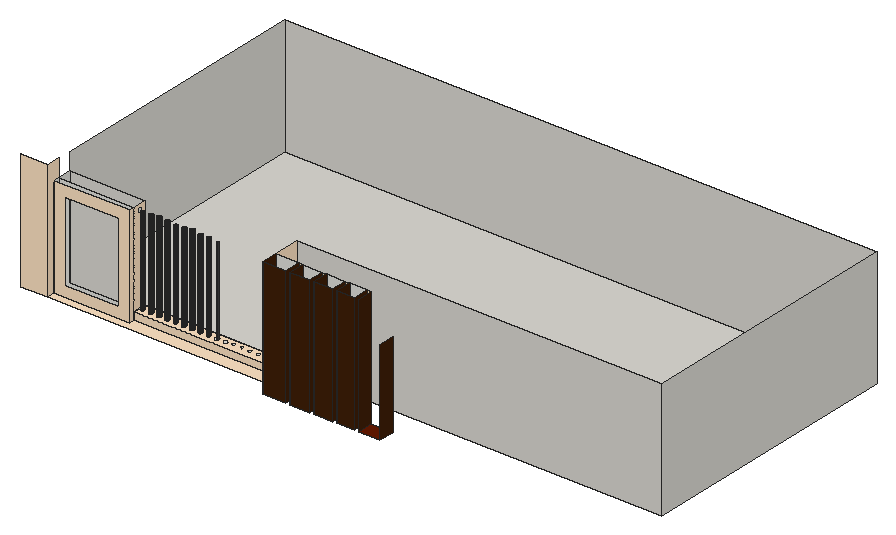
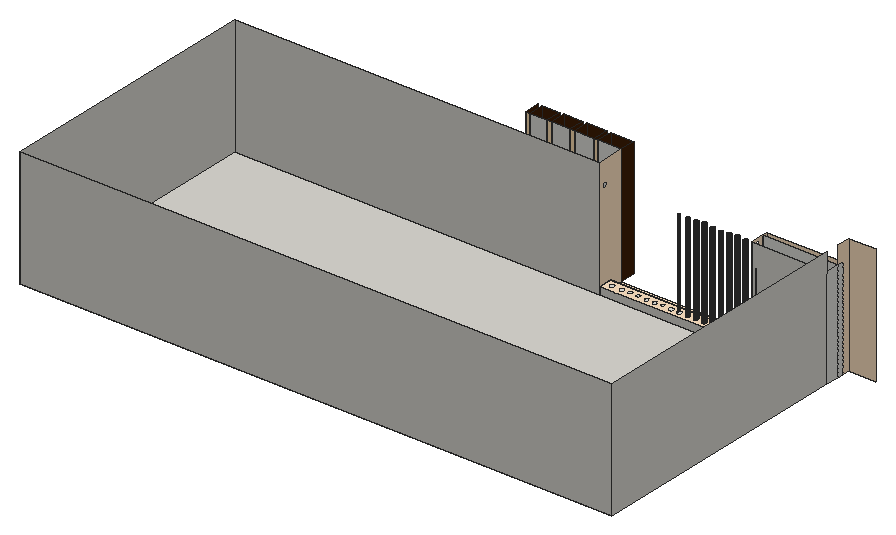
# SketchUp Ruby script. Lengths in inches.
U = 1.inch
M = Sketchup.active_model
def pt(a) = Geom::Point3d.new(a.map { |v| v * U })
def face(e, loops, mat)
  f = e.add_face(loops[0].map { |a| pt(a) })
  loops[1..].each { |l| e.add_face(l.map { |a| pt(a) }).erase! }
  f.material = f.back_material = mat if mat
  f
end
# faces: each face lists its corners as indices into pts; further lists are holes
def faces(e, pts, list, mat = nil) = list.each { |f| face(e, (f[0].is_a?(Array) ? f : [f]).map { |l| l.map { |i| pts[i] } }, mat) }
# xy, xz, yz: faces in a plane at the given z, y or x. An outline is a flat list of corners, or four numbers for a rectangle; further outlines are holes
def ring(l) = l.size == 4 ? [[l[0], l[1]], [l[2], l[1]], [l[2], l[3]], [l[0], l[3]]] : l.each_slice(2).to_a
def flat(e, list, mat, &to3) = list.each { |f| face(e, (f[0].is_a?(Array) ? f : [f]).map { |l| ring(l).map { |u, v| to3.(u, v) } }, mat) }
def xy(e, z, list, mat = nil) = flat(e, list, mat) { |x, y| [x, y, z] }
def xz(e, y, list, mat = nil) = flat(e, list, mat) { |x, z| [x, y, z] }
def yz(e, x, list, mat = nil) = flat(e, list, mat) { |y, z| [x, y, z] }
def lines(e, pts, list) = list.each { |a, b| e.add_line(pt(pts[a]), pt(pts[b])) }
# prism: a flat outline (further loops are holes) pulled along v
def prism(e, loops, v, mat = nil)
  f = face(e, loops, mat); d = Geom::Vector3d.new(v.map { |x| x * U })
  f.pushpull(f.normal.samedirection?(d) ? d.length : -d.length)
end
def box(e, o, s, mat = nil) = prism(e, [[o, [o[0] + s[0], o[1], o[2]], [o[0] + s[0], o[1] + s[1], o[2]], [o[0], o[1] + s[1], o[2]]]], [0, 0, s[2]], mat)
def at(x, y, z, deg = 0) = Geom::Transformation.translation(pt([x, y, z])) * Geom::Transformation.rotation(ORIGIN, Z_AXIS, deg.degrees)
def axes(o, x, y, z) = Geom::Transformation.new([*x, 0, *y, 0, *z, 0, *pt(o).to_a, 1])
def part(name) = M.definitions.add(name)
# library, detail: a bought-in or finely detailed component or shape, given as its bounding box
def library(name, o, s) = part(name).tap { |d| box(d.entities, o, s) }
def detail(e, o, s) = box(e.add_group.entities, o, s)
def put(e, d, t, mat = nil) = e.add_instance(d, t).tap { |i| i.material = mat if mat }
def group(e, t, mat = nil) = e.add_group.tap { |g| g.transformation = t; g.material = mat if mat }.entities
root = M.entities
M.materials.add("[0012_Bisque]").color = [255, 228, 196]
M.materials.add("[0043_SaddleBrown]").color = [63, 31, 8]
M.materials.add("[Color B08]").color = [102, 25, 0]
M.materials.add("[Color M07]").color = [58, 58, 58]
M.materials.add("[Formica Beige]").color = [255, 225, 180]
M.materials.add("[Terrazzo Tile Light]").color = [219, 217, 210]
xy(root,289.4375,[[20.26,180.33,76.27,184.58],[20.26,184.58,76.27,194.72],[76.27,184.58,189.35,194.72]])
xy(root,289.4375,[[20.26,174.45,189.35,174.45,189.35,184.58,76.27,184.58,76.27,180.33,20.26,180.33]],"[0012_Bisque]")
xy(root,289.4375,[[189.35,162.83,206.61,174.45],[209.66,162.83,224.17,174.45],[227.22,162.83,241.23,174.45],[244.28,162.83,257.3,174.45],[260.36,162.83,276.43,174.45]],"[Color B08]")
xy(root,289.4375,[[20.26,194.72,459.74,394.19]],"[Terrazzo Tile Light]")
xy(root,295,[[78.76,188.34,78.4,188.39,78.07,188.53,77.78,188.75,77.56,189.03,77.43,189.36,77.38,189.72,77.43,190.07,77.56,190.41,77.78,190.69,78.07,190.91,78.4,191.05,78.76,191.09,79.11,191.05,79.44,190.91,79.73,190.69,79.95,190.41,80.08,190.07,80.13,189.72,80.08,189.36,79.95,189.03,79.73,188.75,79.44,188.53,79.11,188.39],[84.88,188.34,84.52,188.39,84.19,188.53,83.91,188.75,83.69,189.03,83.55,189.36,83.51,189.72,83.55,190.07,83.69,190.41,83.91,190.69,84.19,190.91,84.52,191.05,84.88,191.09,85.24,191.05,85.57,190.91,85.85,190.69,86.07,190.41,86.21,190.07,86.26,189.72,86.21,189.36,86.07,189.03,85.85,188.75,85.57,188.53,85.24,188.39],[91.01,188.34,90.65,188.39,90.32,188.53,90.03,188.75,89.81,189.03,89.68,189.36,89.63,189.72,89.68,190.07,89.81,190.41,90.03,190.69,90.32,190.91,90.65,191.05,91.01,191.09,91.36,191.05,91.69,190.91,91.98,190.69,92.2,190.41,92.33,190.07,92.38,189.72,92.33,189.36,92.2,189.03,91.98,188.75,91.69,188.53,91.36,188.39],[97.13,188.34,96.77,188.39,96.44,188.53,96.16,188.75,95.94,189.03,95.8,189.36,95.76,189.72,95.8,190.07,95.94,190.41,96.16,190.69,96.44,190.91,96.77,191.05,97.13,191.09,97.49,191.05,97.82,190.91,98.1,190.69,98.32,190.41,98.46,190.07,98.51,189.72,98.46,189.36,98.32,189.03,98.1,188.75,97.82,188.53,97.49,188.39],[103.26,188.34,102.9,188.39,102.57,188.53,102.28,188.75,102.06,189.03,101.93,189.36,101.88,189.72,101.93,190.07,102.06,190.41,102.28,190.69,102.57,190.91,102.9,191.05,103.26,191.09,103.61,191.05,103.94,190.91,104.23,190.69,104.45,190.41,104.58,190.07,104.63,189.72,104.58,189.36,104.45,189.03,104.23,188.75,103.94,188.53,103.61,188.39],
  [109.38,188.34,109.02,188.39,108.69,188.53,108.41,188.75,108.19,189.03,108.05,189.36,108.01,189.72,108.05,190.07,108.19,190.41,108.41,190.69,108.69,190.91,109.02,191.05,109.38,191.09,109.74,191.05,110.07,190.91,110.35,190.69,110.57,190.41,110.71,190.07,110.76,189.72,110.71,189.36,110.57,189.03,110.35,188.75,110.07,188.53,109.74,188.39],[115.51,188.34,115.15,188.39,114.82,188.53,114.53,188.75,114.31,189.03,114.18,189.36,114.13,189.72,114.18,190.07,114.31,190.41,114.53,190.69,114.82,190.91,115.15,191.05,115.51,191.09,115.86,191.05,116.19,190.91,116.48,190.69,116.7,190.41,116.83,190.07,116.88,189.72,116.83,189.36,116.7,189.03,116.48,188.75,116.19,188.53,115.86,188.39],[121.63,188.34,121.27,188.39,120.94,188.53,120.66,188.75,120.44,189.03,120.3,189.36,120.26,189.72,120.3,190.07,120.44,190.41,120.66,190.69,120.94,190.91,121.27,191.05,121.63,191.09,121.99,191.05,122.32,190.91,122.6,190.69,122.82,190.41,122.96,190.07,123.01,189.72,122.96,189.36,122.82,189.03,122.6,188.75,122.32,188.53,121.99,188.39],[127.76,188.34,127.4,188.39,127.07,188.53,126.78,188.75,126.56,189.03,126.43,189.36,126.38,189.72,126.43,190.07,126.56,190.41,126.78,190.69,127.07,190.91,127.4,191.05,127.76,191.09,128.11,191.05,128.44,190.91,128.73,190.69,128.95,190.41,129.08,190.07,129.13,189.72,129.08,189.36,128.95,189.03,128.73,188.75,128.44,188.53,128.11,188.39],[133.88,188.34,133.52,188.39,133.19,188.53,132.91,188.75,132.69,189.03,132.55,189.36,132.51,189.72,132.55,190.07,132.69,190.41,132.91,190.69,133.19,190.91,133.52,191.05,133.88,191.09,134.24,191.05,134.57,190.91,134.85,190.69,135.07,190.41,135.21,190.07,135.26,189.72,135.21,189.36,135.07,189.03,134.85,188.75,134.57,188.53,134.24,188.39],
  [140.01,188.34,139.65,188.39,139.32,188.53,139.03,188.75,138.81,189.03,138.68,189.36,138.63,189.72,138.68,190.07,138.81,190.41,139.03,190.69,139.32,190.91,139.65,191.05,140.01,191.09,140.36,191.05,140.69,190.91,140.98,190.69,141.2,190.41,141.33,190.07,141.38,189.72,141.33,189.36,141.2,189.03,140.98,188.75,140.69,188.53,140.36,188.39],[146.13,188.34,145.77,188.39,145.44,188.53,145.16,188.75,144.94,189.03,144.8,189.36,144.76,189.72,144.8,190.07,144.94,190.41,145.16,190.69,145.44,190.91,145.77,191.05,146.13,191.09,146.49,191.05,146.82,190.91,147.1,190.69,147.32,190.41,147.46,190.07,147.51,189.72,147.46,189.36,147.32,189.03,147.1,188.75,146.82,188.53,146.49,188.39],[152.26,188.34,151.9,188.39,151.57,188.53,151.28,188.75,151.06,189.03,150.93,189.36,150.88,189.72,150.93,190.07,151.06,190.41,151.28,190.69,151.57,190.91,151.9,191.05,152.26,191.09,152.61,191.05,152.94,190.91,153.23,190.69,153.45,190.41,153.58,190.07,153.63,189.72,153.58,189.36,153.45,189.03,153.23,188.75,152.94,188.53,152.61,188.39],[158.38,188.34,158.02,188.39,157.69,188.53,157.41,188.75,157.19,189.03,157.05,189.36,157.01,189.72,157.05,190.07,157.19,190.41,157.41,190.69,157.69,190.91,158.02,191.05,158.38,191.09,158.74,191.05,159.07,190.91,159.35,190.69,159.57,190.41,159.71,190.07,159.76,189.72,159.71,189.36,159.57,189.03,159.35,188.75,159.07,188.53,158.74,188.39],[164.51,188.34,164.15,188.39,163.82,188.53,163.53,188.75,163.31,189.03,163.18,189.36,163.13,189.72,163.18,190.07,163.31,190.41,163.53,190.69,163.82,190.91,164.15,191.05,164.51,191.09,164.86,191.05,165.19,190.91,165.48,190.69,165.7,190.41,165.83,190.07,165.88,189.72,165.83,189.36,165.7,189.03,165.48,188.75,165.19,188.53,164.86,188.39],
  [170.63,188.34,170.27,188.39,169.94,188.53,169.66,188.75,169.44,189.03,169.3,189.36,169.26,189.72,169.3,190.07,169.44,190.41,169.66,190.69,169.94,190.91,170.27,191.05,170.63,191.09,170.99,191.05,171.32,190.91,171.6,190.69,171.82,190.41,171.96,190.07,172.01,189.72,171.96,189.36,171.82,189.03,171.6,188.75,171.32,188.53,170.99,188.39],[176.82,188.34,176.46,188.39,176.13,188.53,175.85,188.75,175.63,189.03,175.49,189.36,175.44,189.72,175.49,190.07,175.63,190.41,175.85,190.69,176.13,190.91,176.46,191.05,176.82,191.09,177.17,191.05,177.51,190.91,177.79,190.69,178.01,190.41,178.15,190.07,178.19,189.72,178.15,189.36,178.01,189.03,177.79,188.75,177.51,188.53,177.17,188.39],[184.01,188.34,183.65,188.39,183.32,188.53,183.03,188.75,182.81,189.03,182.68,189.36,182.63,189.72,182.68,190.07,182.81,190.41,183.03,190.69,183.32,190.91,183.65,191.05,184.01,191.09,184.36,191.05,184.69,190.91,184.98,190.69,185.2,190.41,185.33,190.07,185.38,189.72,185.33,189.36,185.2,189.03,184.98,188.75,184.69,188.53,184.36,188.39]])
xy(root,295,[[[76.27,184.58,189.35,194.72],[78.76,188.34,78.4,188.39,78.07,188.53,77.78,188.75,77.56,189.03,77.43,189.36,77.38,189.72,77.43,190.07,77.56,190.41,77.78,190.69,78.07,190.91,78.4,191.05,78.76,191.09,79.11,191.05,79.44,190.91,79.73,190.69,79.95,190.41,80.08,190.07,80.13,189.72,80.08,189.36,79.95,189.03,79.73,188.75,79.44,188.53,79.11,188.39],[84.88,188.34,84.52,188.39,84.19,188.53,83.91,188.75,83.69,189.03,83.55,189.36,83.51,189.72,83.55,190.07,83.69,190.41,83.91,190.69,84.19,190.91,84.52,191.05,84.88,191.09,85.24,191.05,85.57,190.91,85.85,190.69,86.07,190.41,86.21,190.07,86.26,189.72,86.21,189.36,86.07,189.03,85.85,188.75,85.57,188.53,85.24,188.39],[91.01,188.34,90.65,188.39,90.32,188.53,90.03,188.75,89.81,189.03,89.68,189.36,89.63,189.72,89.68,190.07,89.81,190.41,90.03,190.69,90.32,190.91,90.65,191.05,91.01,191.09,91.36,191.05,91.69,190.91,91.98,190.69,92.2,190.41,92.33,190.07,92.38,189.72,92.33,189.36,92.2,189.03,91.98,188.75,91.69,188.53,91.36,188.39],[97.13,188.34,96.77,188.39,96.44,188.53,96.16,188.75,95.94,189.03,95.8,189.36,95.76,189.72,95.8,190.07,95.94,190.41,96.16,190.69,96.44,190.91,96.77,191.05,97.13,191.09,97.49,191.05,97.82,190.91,98.1,190.69,98.32,190.41,98.46,190.07,98.51,189.72,98.46,189.36,98.32,189.03,98.1,188.75,97.82,188.53,97.49,188.39],[103.26,188.34,102.9,188.39,102.57,188.53,102.28,188.75,102.06,189.03,101.93,189.36,101.88,189.72,101.93,190.07,102.06,190.41,102.28,190.69,102.57,190.91,102.9,191.05,103.26,191.09,103.61,191.05,103.94,190.91,104.23,190.69,104.45,190.41,104.58,190.07,104.63,189.72,104.58,189.36,104.45,189.03,104.23,188.75,103.94,188.53,103.61,188.39],[109.38,188.34,109.02,188.39,108.69,188.53,108.41,188.75,108.19,189.03,108.05,189.36,108.01,189.72,108.05,190.07,108.19,190.41,108.41,190.69,108.69,190.91,109.02,191.05,109.38,191.09,109.74,191.05,110.07,190.91,110.35,190.69,110.57,190.41,110.71,190.07,110.76,189.72,110.71,189.36,110.57,189.03,110.35,188.75,110.07,188.53,109.74,188.39],[115.51,188.34,115.15,188.39,114.82,188.53,114.53,188.75,114.31,189.03,114.18,189.36,114.13,189.72,114.18,190.07,114.31,190.41,114.53,190.69,114.82,190.91,115.15,191.05,115.51,191.09,115.86,191.05,116.19,190.91,116.48,190.69,116.7,190.41,116.83,190.07,116.88,189.72,116.83,189.36,116.7,189.03,116.48,188.75,116.19,188.53,115.86,188.39],[121.63,188.34,121.27,188.39,120.94,188.53,120.66,188.75,120.44,189.03,120.3,189.36,120.26,189.72,120.3,190.07,120.44,190.41,120.66,190.69,120.94,190.91,121.27,191.05,121.63,191.09,121.99,191.05,122.32,190.91,122.6,190.69,122.82,190.41,122.96,190.07,123.01,189.72,122.96,189.36,122.82,189.03,122.6,188.75,122.32,188.53,121.99,188.39],[127.76,188.34,127.4,188.39,127.07,188.53,126.78,188.75,126.56,189.03,126.43,189.36,126.38,189.72,126.43,190.07,126.56,190.41,126.78,190.69,127.07,190.91,127.4,191.05,127.76,191.09,128.11,191.05,128.44,190.91,128.73,190.69,128.95,190.41,129.08,190.07,129.13,189.72,129.08,189.36,128.95,189.03,128.73,188.75,128.44,188.53,128.11,188.39],[133.88,188.34,133.52,188.39,133.19,188.53,132.91,188.75,132.69,189.03,132.55,189.36,132.51,189.72,132.55,190.07,132.69,190.41,132.91,190.69,133.19,190.91,133.52,191.05,133.88,191.09,134.24,191.05,134.57,190.91,134.85,190.69,135.07,190.41,135.21,190.07,135.26,189.72,135.21,189.36,135.07,189.03,134.85,188.75,134.57,188.53,134.24,188.39],[140.01,188.34,139.65,188.39,139.32,188.53,139.03,188.75,138.81,189.03,138.68,189.36,138.63,189.72,138.68,190.07,138.81,190.41,139.03,190.69,139.32,190.91,139.65,191.05,140.01,191.09,140.36,191.05,140.69,190.91,140.98,190.69,141.2,190.41,141.33,190.07,141.38,189.72,141.33,189.36,141.2,189.03,140.98,188.75,140.69,188.53,140.36,188.39],[146.13,188.34,145.77,188.39,145.44,188.53,145.16,188.75,144.94,189.03,144.8,189.36,144.76,189.72,144.8,190.07,144.94,190.41,145.16,190.69,145.44,190.91,145.77,191.05,146.13,191.09,146.49,191.05,146.82,190.91,147.1,190.69,147.32,190.41,147.46,190.07,147.51,189.72,147.46,189.36,147.32,189.03,147.1,188.75,146.82,188.53,146.49,188.39],[152.26,188.34,151.9,188.39,151.57,188.53,151.28,188.75,151.06,189.03,150.93,189.36,150.88,189.72,150.93,190.07,151.06,190.41,151.28,190.69,151.57,190.91,151.9,191.05,152.26,191.09,152.61,191.05,152.94,190.91,153.23,190.69,153.45,190.41,153.58,190.07,153.63,189.72,153.58,189.36,153.45,189.03,153.23,188.75,152.94,188.53,152.61,188.39],[158.38,188.34,158.02,188.39,157.69,188.53,157.41,188.75,157.19,189.03,157.05,189.36,157.01,189.72,157.05,190.07,157.19,190.41,157.41,190.69,157.69,190.91,158.02,191.05,158.38,191.09,158.74,191.05,159.07,190.91,159.35,190.69,159.57,190.41,159.71,190.07,159.76,189.72,159.71,189.36,159.57,189.03,159.35,188.75,159.07,188.53,158.74,188.39],[164.51,188.34,164.15,188.39,163.82,188.53,163.53,188.75,163.31,189.03,163.18,189.36,163.13,189.72,163.18,190.07,163.31,190.41,163.53,190.69,163.82,190.91,164.15,191.05,164.51,191.09,164.86,191.05,165.19,190.91,165.48,190.69,165.7,190.41,165.83,190.07,165.88,189.72,165.83,189.36,165.7,189.03,165.48,188.75,165.19,188.53,164.86,188.39],[170.63,188.34,170.27,188.39,169.94,188.53,169.66,188.75,169.44,189.03,169.3,189.36,169.26,189.72,169.3,190.07,169.44,190.41,169.66,190.69,169.94,190.91,170.27,191.05,170.63,191.09,170.99,191.05,171.32,190.91,171.6,190.69,171.82,190.41,171.96,190.07,172.01,189.72,171.96,189.36,171.82,189.03,171.6,188.75,171.32,188.53,170.99,188.39],[176.82,188.34,176.46,188.39,176.13,188.53,175.85,188.75,175.63,189.03,175.49,189.36,175.44,189.72,175.49,190.07,175.63,190.41,175.85,190.69,176.13,190.91,176.46,191.05,176.82,191.09,177.17,191.05,177.51,190.91,177.79,190.69,178.01,190.41,178.15,190.07,178.19,189.72,178.15,189.36,178.01,189.03,177.79,188.75,177.51,188.53,177.17,188.39],[184.01,188.34,183.65,188.39,183.32,188.53,183.03,188.75,182.81,189.03,182.68,189.36,182.63,189.72,182.68,190.07,182.81,190.41,183.03,190.69,183.32,190.91,183.65,191.05,184.01,191.09,184.36,191.05,184.69,190.91,184.98,190.69,185.2,190.41,185.33,190.07,185.38,189.72,185.33,189.36,185.2,189.03,184.98,188.75,184.69,188.53,184.36,188.39]]],"[0012_Bisque]")
xz(root,162.83,[[189.35,289.4375,206.61,377.375],[209.66,289.4375,224.17,377.375],[227.22,289.4375,241.23,377.375],[244.28,289.4375,257.3,377.375]],"[0043_SaddleBrown]")
xz(root,174.45,[[189.35,289.4375,206.61,377.375],[209.66,289.4375,224.17,377.375],[227.22,289.4375,241.23,377.375],[244.28,289.4375,257.3,377.375]])
xz(root,174.45,[[0,289.4375,20.26,377.375]],"[0012_Bisque]")
xz(root,174.45,[[206.61,289.4375,209.66,377.375],[224.17,289.4375,227.22,377.375],[241.23,289.4375,244.28,377.375],[257.3,289.4375,260.36,377.375]],"[Formica Beige]")
xz(root,180.33,[[[20.26,289.4375,76.27,364.375],[28.1875,297.36,68.35,356.45]]],"[0012_Bisque]")
xz(root,184.58,[[[20.26,289.4375,76.27,364.375],[28.1875,297.36,68.35,356.45]]])
xz(root,184.58,[[76.27,289.4375,189.35,295]],"[0012_Bisque]")
xz(root,194.72,[[20.26,289.4375,76.27,364.375],[76.27,289.4375,189.35,295],[189.35,289.4375,459.74,377.375]],"[Terrazzo Tile Light]")
xz(root,394.19,[[20.26,289.4375,459.74,377.375]],"[Terrazzo Tile Light]")
yz(root,20.26,[[180.33,289.4375,184.58,364.375],[184.58,289.4375,194.72,364.375]])
yz(root,20.26,[[174.45,289.4375,180.33,289.4375,180.33,364.375,184.58,364.375,184.58,377.375,174.45,377.375]],"[0012_Bisque]")
yz(root,20.26,[[194.72,289.4375,394.19,377.375]],"[Terrazzo Tile Light]")
yz(root,76.27,[[184.58,289.4375,194.72,295]])
yz(root,76.27,[[180.33,289.4375,184.58,364.375],[[184.58,295,194.72,364.375],[189.8125,358.43,189.28,358.5,188.78,358.7,188.35,359.03,188.02,359.46,187.82,359.95,187.75,360.49,187.82,361.02,188.02,361.52,188.35,361.95,188.78,362.27,189.28,362.48,189.8125,362.55,190.34,362.48,190.84,362.27,191.27,361.95,191.6,361.52,191.8,361.02,191.875,360.49,191.8,359.95,191.6,359.46,191.27,359.03,190.84,358.7,190.34,358.5]]],"[0012_Bisque]")
yz(root,189.35,[[184.58,289.4375,194.72,295]])
yz(root,189.35,[[[174.45,289.4375,174.45,377.375,194.72,377.375,194.72,295,184.58,295,184.58,289.4375],[189.8125,358.43,190.34,358.5,190.84,358.7,191.27,359.03,191.6,359.46,191.8,359.95,191.875,360.49,191.8,361.02,191.6,361.52,191.27,361.95,190.84,362.27,190.34,362.48,189.8125,362.55,189.28,362.48,188.78,362.27,188.35,361.95,188.02,361.52,187.82,361.02,187.75,360.49,187.82,359.95,188.02,359.46,188.35,359.03,188.78,358.7,189.28,358.5]]],"[0012_Bisque]")
yz(root,189.35,[[162.83,289.4375,174.45,377.375]],"[0043_SaddleBrown]")
yz(root,206.61,[[162.83,289.4375,174.45,377.375]],"[0043_SaddleBrown]")
yz(root,209.66,[[162.83,289.4375,174.45,377.375]],"[0043_SaddleBrown]")
yz(root,224.17,[[162.83,289.4375,174.45,377.375]],"[0043_SaddleBrown]")
yz(root,227.22,[[162.83,289.4375,174.45,377.375]],"[0043_SaddleBrown]")
yz(root,241.23,[[162.83,289.4375,174.45,377.375]],"[0043_SaddleBrown]")
yz(root,244.28,[[162.83,289.4375,174.45,377.375]],"[0043_SaddleBrown]")
yz(root,257.3,[[162.83,289.4375,174.45,377.375]],"[0043_SaddleBrown]")
yz(root,260.36,[[162.83,289.4375,174.45,377.375]],"[0043_SaddleBrown]")
yz(root,276.43,[[162.83,289.4375,174.45,352.96]],"[0043_SaddleBrown]")
yz(root,459.74,[[194.72,289.4375,394.19,377.375]],"[Terrazzo Tile Light]")
p = [[78.4,188.39,295],[78.76,188.34,295],[78.76,188.34,360.125],[78.4,188.39,360.125],[79.11,188.39,295],[79.11,188.39,360.125],
  [84.52,188.39,295],[84.88,188.34,295],[84.88,188.34,360.1875],[84.52,188.39,360.1875],[85.24,188.39,295],[85.24,188.39,360.1875],
  [90.65,188.39,295],[91.01,188.34,295],[91.01,188.34,361.02],[90.65,188.39,361.02],[91.36,188.39,295],[91.36,188.39,361.02],
  [96.77,188.39,295],[97.13,188.34,295],[97.13,188.34,360.3125],[96.77,188.39,360.3125],[97.49,188.39,295],[97.49,188.39,360.3125],
  [102.9,188.39,295],[103.26,188.34,295],[103.26,188.34,359.5625],[102.9,188.39,359.5625],[103.61,188.39,295],[103.61,188.39,359.5625],
  [109.02,188.39,295],[109.38,188.34,295],[109.38,188.34,359.9375],[109.02,188.39,359.9375],[109.74,188.39,295],[109.74,188.39,359.9375],
  [115.15,188.39,295],[115.51,188.34,295],[115.51,188.34,361.02],[115.15,188.39,361.02],[115.86,188.39,295],[115.86,188.39,361.02],
  [121.27,188.39,295],[121.63,188.34,295],[121.63,188.34,359.95],[121.27,188.39,359.95],[121.99,188.39,295],[121.99,188.39,359.95],
  [127.4,188.39,295],[127.76,188.34,295],[127.76,188.34,359.9375],[127.4,188.39,359.9375],[128.11,188.39,295],[128.11,188.39,359.9375],
  [78.07,188.53,295],[78.07,188.53,360.125],[79.44,188.53,295],[79.44,188.53,360.125],[84.19,188.53,295],[84.19,188.53,360.1875],
  [85.57,188.53,295],[85.57,188.53,360.1875],[90.32,188.53,295],[90.32,188.53,361.02],[91.69,188.53,295],[91.69,188.53,361.02],
  [96.44,188.53,295],[96.44,188.53,360.3125],[97.82,188.53,295],[97.82,188.53,360.3125],[102.57,188.53,295],[102.57,188.53,359.5625],
  [103.94,188.53,295],[103.94,188.53,359.5625],[108.69,188.53,295],[108.69,188.53,359.9375],[110.07,188.53,295],[110.07,188.53,359.9375],
  [114.82,188.53,295],[114.82,188.53,361.02],[116.19,188.53,295],[116.19,188.53,361.02],[120.94,188.53,295],[120.94,188.53,359.95],
  [122.32,188.53,295],[122.32,188.53,359.95],[127.07,188.53,295],[127.07,188.53,359.9375],[128.44,188.53,295],[128.44,188.53,359.9375],
  [77.78,188.75,295],[77.78,188.75,360.125],[79.73,188.75,295],[79.73,188.75,360.125],[83.91,188.75,295],[83.91,188.75,360.1875],
  [85.85,188.75,295],[85.85,188.75,360.1875],[90.03,188.75,295],[90.03,188.75,361.02],[91.98,188.75,295],[91.98,188.75,361.02],
  [96.16,188.75,295],[96.16,188.75,360.3125],[98.1,188.75,295],[98.1,188.75,360.3125],[102.28,188.75,295],[102.28,188.75,359.5625],
  [104.23,188.75,295],[104.23,188.75,359.5625],[108.41,188.75,295],[108.41,188.75,359.9375],[110.35,188.75,295],[110.35,188.75,359.9375],
  [114.53,188.75,295],[114.53,188.75,361.02],[116.48,188.75,295],[116.48,188.75,361.02],[120.66,188.75,295],[120.66,188.75,359.95],
  [122.6,188.75,295],[122.6,188.75,359.95],[126.78,188.75,295],[126.78,188.75,359.9375],[128.73,188.75,295],[128.73,188.75,359.9375],
  [134.57,188.53,295],[134.85,188.75,295],[134.85,188.75,360],[134.57,188.53,360],[77.56,189.03,295],[77.56,189.03,360.125],
  [79.95,189.03,295],[79.95,189.03,360.125],[83.69,189.03,295],[83.69,189.03,360.1875],[86.07,189.03,295],[86.07,189.03,360.1875],
  [89.81,189.03,295],[89.81,189.03,361.02],[92.2,189.03,295],[92.2,189.03,361.02],[95.94,189.03,295],[95.94,189.03,360.3125],
  [98.32,189.03,295],[98.32,189.03,360.3125],[102.06,189.03,295],[102.06,189.03,359.5625],[104.45,189.03,295],[104.45,189.03,359.5625],
  [108.19,189.03,295],[108.19,189.03,359.9375],[110.57,189.03,295],[110.57,189.03,359.9375],[114.31,189.03,295],[114.31,189.03,361.02],
  [116.7,189.03,295],[116.7,189.03,361.02],[120.44,189.03,295],[120.44,189.03,359.95],[122.82,189.03,295],[122.82,189.03,359.95],
  [126.56,189.03,295],[126.56,189.03,359.9375],[128.95,189.03,295],[128.95,189.03,359.9375],[135.07,189.03,295],[135.07,189.03,360],
  [77.43,189.36,295],[77.43,189.36,360.125],[80.08,189.36,295],[80.08,189.36,360.125],[83.55,189.36,295],[83.55,189.36,360.1875],
  [86.21,189.36,295],[86.21,189.36,360.1875],[89.68,189.36,295],[89.68,189.36,361.02],[92.33,189.36,295],[92.33,189.36,361.02],
  [95.8,189.36,295],[95.8,189.36,360.3125],[98.46,189.36,295],[98.46,189.36,360.3125],[101.93,189.36,295],[101.93,189.36,359.5625],
  [104.58,189.36,295],[104.58,189.36,359.5625],[108.05,189.36,295],[108.05,189.36,359.9375],[110.71,189.36,295],[110.71,189.36,359.9375],
  [114.18,189.36,295],[114.18,189.36,361.02],[116.83,189.36,295],[116.83,189.36,361.02],[120.3,189.36,295],[120.3,189.36,359.95],
  [122.96,189.36,295],[122.96,189.36,359.95],[126.43,189.36,295],[126.43,189.36,359.9375],[129.08,189.36,295],[129.08,189.36,359.9375],
  [135.21,189.36,295],[135.21,189.36,360],[77.38,189.72,295],[77.38,189.72,360.125],[80.13,189.72,295],[80.13,189.72,360.125],
  [83.51,189.72,295],[83.51,189.72,360.1875],[86.26,189.72,295],[86.26,189.72,360.1875],[89.63,189.72,295],[89.63,189.72,361.02],
  [92.38,189.72,295],[92.38,189.72,361.02],[95.76,189.72,295],[95.76,189.72,360.3125],[98.51,189.72,295],[98.51,189.72,360.3125],
  [101.88,189.72,295],[101.88,189.72,359.5625],[104.63,189.72,295],[104.63,189.72,359.5625],[108.01,189.72,295],[108.01,189.72,359.9375],
  [110.76,189.72,295],[110.76,189.72,359.9375],[114.13,189.72,295],[114.13,189.72,361.02],[116.88,189.72,295],[116.88,189.72,361.02],
  [120.26,189.72,295],[120.26,189.72,359.95],[123.01,189.72,295],[123.01,189.72,359.95],[126.38,189.72,295],[126.38,189.72,359.9375],
  [129.13,189.72,295],[129.13,189.72,359.9375],[77.43,190.07,295],[77.43,190.07,360.125],[80.08,190.07,295],[80.08,190.07,360.125],
  [83.55,190.07,295],[83.55,190.07,360.1875],[86.21,190.07,295],[86.21,190.07,360.1875],[89.68,190.07,295],[89.68,190.07,361.02],
  [92.33,190.07,295],[92.33,190.07,361.02],[95.8,190.07,295],[95.8,190.07,360.3125],[98.46,190.07,295],[98.46,190.07,360.3125],
  [101.93,190.07,295],[101.93,190.07,359.5625],[104.58,190.07,295],[104.58,190.07,359.5625],[108.05,190.07,295],[108.05,190.07,359.9375],
  [110.71,190.07,295],[110.71,190.07,359.9375],[114.18,190.07,295],[114.18,190.07,361.02],[116.83,190.07,295],[116.83,190.07,361.02],
  [120.3,190.07,295],[120.3,190.07,359.95],[122.96,190.07,295],[122.96,190.07,359.95],[126.43,190.07,295],[126.43,190.07,359.9375],
  [129.08,190.07,295],[129.08,190.07,359.9375],[77.56,190.41,295],[77.56,190.41,360.125],[79.95,190.41,295],[79.95,190.41,360.125],
  [83.69,190.41,295],[83.69,190.41,360.1875],[86.07,190.41,295],[86.07,190.41,360.1875],[89.81,190.41,295],[89.81,190.41,361.02],
  [92.2,190.41,295],[92.2,190.41,361.02],[95.94,190.41,295],[95.94,190.41,360.3125],[98.32,190.41,295],[98.32,190.41,360.3125],
  [102.06,190.41,295],[102.06,190.41,359.5625],[104.45,190.41,295],[104.45,190.41,359.5625],[108.19,190.41,295],[108.19,190.41,359.9375],
  [110.57,190.41,295],[110.57,190.41,359.9375],[114.31,190.41,295],[114.31,190.41,361.02],[116.7,190.41,295],[116.7,190.41,361.02],
  [120.44,190.41,295],[120.44,190.41,359.95],[122.82,190.41,295],[122.82,190.41,359.95],[126.56,190.41,295],[126.56,190.41,359.9375],
  [128.95,190.41,295],[128.95,190.41,359.9375],[77.78,190.69,295],[77.78,190.69,360.125],[79.73,190.69,295],[79.73,190.69,360.125],
  [83.91,190.69,295],[83.91,190.69,360.1875],[85.85,190.69,295],[85.85,190.69,360.1875],[90.03,190.69,295],[90.03,190.69,361.02],
  [91.98,190.69,295],[91.98,190.69,361.02],[96.16,190.69,295],[96.16,190.69,360.3125],[98.1,190.69,295],[98.1,190.69,360.3125],
  [102.28,190.69,295],[102.28,190.69,359.5625],[104.23,190.69,295],[104.23,190.69,359.5625],[108.41,190.69,295],[108.41,190.69,359.9375],
  [110.35,190.69,295],[110.35,190.69,359.9375],[114.53,190.69,295],[114.53,190.69,361.02],[116.48,190.69,295],[116.48,190.69,361.02],
  [120.66,190.69,295],[120.66,190.69,359.95],[122.6,190.69,295],[122.6,190.69,359.95],[126.78,190.69,295],[126.78,190.69,359.9375],
  [128.73,190.69,295],[128.73,190.69,359.9375],[78.07,190.91,295],[78.07,190.91,360.125],[79.44,190.91,295],[79.44,190.91,360.125],
  [84.19,190.91,295],[84.19,190.91,360.1875],[85.57,190.91,295],[85.57,190.91,360.1875],[90.32,190.91,295],[90.32,190.91,361.02],
  [91.69,190.91,295],[91.69,190.91,361.02],[96.44,190.91,295],[96.44,190.91,360.3125],[97.82,190.91,295],[97.82,190.91,360.3125],
  [102.57,190.91,295],[102.57,190.91,359.5625],[103.94,190.91,295],[103.94,190.91,359.5625],[108.69,190.91,295],[108.69,190.91,359.9375],
  [110.07,190.91,295],[110.07,190.91,359.9375],[114.82,190.91,295],[114.82,190.91,361.02],[116.19,190.91,295],[116.19,190.91,361.02],
  [120.94,190.91,295],[120.94,190.91,359.95],[122.32,190.91,295],[122.32,190.91,359.95],[127.07,190.91,295],[127.07,190.91,359.9375],
  [128.44,190.91,295],[128.44,190.91,359.9375],[78.4,191.05,295],[78.4,191.05,360.125],[79.11,191.05,295],[79.11,191.05,360.125],
  [84.52,191.05,295],[84.52,191.05,360.1875],[85.24,191.05,295],[85.24,191.05,360.1875],[90.65,191.05,295],[90.65,191.05,361.02],
  [91.36,191.05,295],[91.36,191.05,361.02],[96.77,191.05,295],[96.77,191.05,360.3125],[97.49,191.05,295],[97.49,191.05,360.3125],
  [102.9,191.05,295],[102.9,191.05,359.5625],[103.61,191.05,295],[103.61,191.05,359.5625],[109.02,191.05,295],[109.02,191.05,359.9375],
  [109.74,191.05,295],[109.74,191.05,359.9375],[115.15,191.05,295],[115.15,191.05,361.02],[115.86,191.05,295],[115.86,191.05,361.02],
  [121.27,191.05,295],[121.27,191.05,359.95],[121.99,191.05,295],[121.99,191.05,359.95],[127.4,191.05,295],[127.4,191.05,359.9375],
  [128.11,191.05,295],[128.11,191.05,359.9375],[78.76,191.09,295],[78.76,191.09,360.125],[84.88,191.09,295],[84.88,191.09,360.1875],
  [91.01,191.09,295],[91.01,191.09,361.02],[97.13,191.09,295],[97.13,191.09,360.3125],[103.26,191.09,295],[103.26,191.09,359.5625],
  [109.38,191.09,295],[109.38,191.09,359.9375],[115.51,191.09,295],[115.51,191.09,361.02],[121.63,191.09,295],[121.63,191.09,359.95],
  [127.76,191.09,295],[127.76,191.09,359.9375]]
faces(root,p,[[0,1,2,3],[1,4,5,2],[6,7,8,9],[7,10,11,8],[12,13,14,15],[13,16,17,14],[18,19,20,21],[19,22,23,20],
  [24,25,26,27],[25,28,29,26],[30,31,32,33],[31,34,35,32],[36,37,38,39],[37,40,41,38],[42,43,44,45],[43,46,47,44],
  [48,49,50,51],[49,52,53,50],[54,0,3,55],[4,56,57,5],[58,6,9,59],[10,60,61,11],[62,12,15,63],[16,64,65,17],
  [66,18,21,67],[22,68,69,23],[70,24,27,71],[28,72,73,29],[74,30,33,75],[34,76,77,35],[78,36,39,79],[40,80,81,41],
  [82,42,45,83],[46,84,85,47],[86,48,51,87],[52,88,89,53],[90,54,55,91],[56,92,93,57],[94,58,59,95],[60,96,97,61],
  [98,62,63,99],[64,100,101,65],[102,66,67,103],[68,104,105,69],[106,70,71,107],[72,108,109,73],[110,74,75,111],[76,112,113,77],
  [114,78,79,115],[80,116,117,81],[118,82,83,119],[84,120,121,85],[122,86,87,123],[88,124,125,89],[126,127,128,129],[130,90,91,131],
  [92,132,133,93],[134,94,95,135],[96,136,137,97],[138,98,99,139],[100,140,141,101],[142,102,103,143],[104,144,145,105],[146,106,107,147],
  [108,148,149,109],[150,110,111,151],[112,152,153,113],[154,114,115,155],[116,156,157,117],[158,118,119,159],[120,160,161,121],[162,122,123,163],
  [124,164,165,125],[127,166,167,128],[168,130,131,169],[132,170,171,133],[172,134,135,173],[136,174,175,137],[176,138,139,177],[140,178,179,141],
  [180,142,143,181],[144,182,183,145],[184,146,147,185],[148,186,187,149],[188,150,151,189],[152,190,191,153],[192,154,155,193],[156,194,195,157],
  [196,158,159,197],[160,198,199,161],[200,162,163,201],[164,202,203,165],[166,204,205,167],[206,168,169,207],[170,208,209,171],[210,172,173,211],
  [174,212,213,175],[214,176,177,215],[178,216,217,179],[218,180,181,219],[182,220,221,183],[222,184,185,223],[186,224,225,187],[226,188,189,227],
  [190,228,229,191],[230,192,193,231],[194,232,233,195],[234,196,197,235],[198,236,237,199],[238,200,201,239],[202,240,241,203],[242,206,207,243],
  [208,244,245,209],[246,210,211,247],[212,248,249,213],[250,214,215,251],[216,252,253,217],[254,218,219,255],[220,256,257,221],[258,222,223,259],
  [224,260,261,225],[262,226,227,263],[228,264,265,229],[266,230,231,267],[232,268,269,233],[270,234,235,271],[236,272,273,237],[274,238,239,275],
  [240,276,277,241],[278,242,243,279],[244,280,281,245],[282,246,247,283],[248,284,285,249],[286,250,251,287],[252,288,289,253],[290,254,255,291],
  [256,292,293,257],[294,258,259,295],[260,296,297,261],[298,262,263,299],[264,300,301,265],[302,266,267,303],[268,304,305,269],[306,270,271,307],
  [272,308,309,273],[310,274,275,311],[276,312,313,277],[314,278,279,315],[280,316,317,281],[318,282,283,319],[284,320,321,285],[322,286,287,323],
  [288,324,325,289],[326,290,291,327],[292,328,329,293],[330,294,295,331],[296,332,333,297],[334,298,299,335],[300,336,337,301],[338,302,303,339],
  [304,340,341,305],[342,306,307,343],[308,344,345,309],[346,310,311,347],[312,348,349,313],[350,314,315,351],[316,352,353,317],[354,318,319,355],
  [320,356,357,321],[358,322,323,359],[324,360,361,325],[362,326,327,363],[328,364,365,329],[366,330,331,367],[332,368,369,333],[370,334,335,371],
  [336,372,373,337],[374,338,339,375],[340,376,377,341],[378,342,343,379],[344,380,381,345],[382,346,347,383],[348,384,385,349],[386,350,351,387],
  [352,388,389,353],[390,354,355,391],[356,392,393,357],[394,358,359,395],[360,396,397,361],[398,362,363,399],[364,400,401,365],[402,366,367,403],
  [368,404,405,369],[406,370,371,407],[372,408,409,373],[410,374,375,411],[376,412,413,377],[414,378,379,415],[380,416,417,381],[418,382,383,419],
  [384,420,421,385],[422,386,387,423],[388,422,423,389],[424,390,391,425],[392,424,425,393],[426,394,395,427],[396,426,427,397],[428,398,399,429],
  [400,428,429,401],[430,402,403,431],[404,430,431,405],[432,406,407,433],[408,432,433,409],[434,410,411,435],[412,434,435,413],[436,414,415,437],
  [416,436,437,417],[438,418,419,439],[420,438,439,421]],"[Color M07]")
